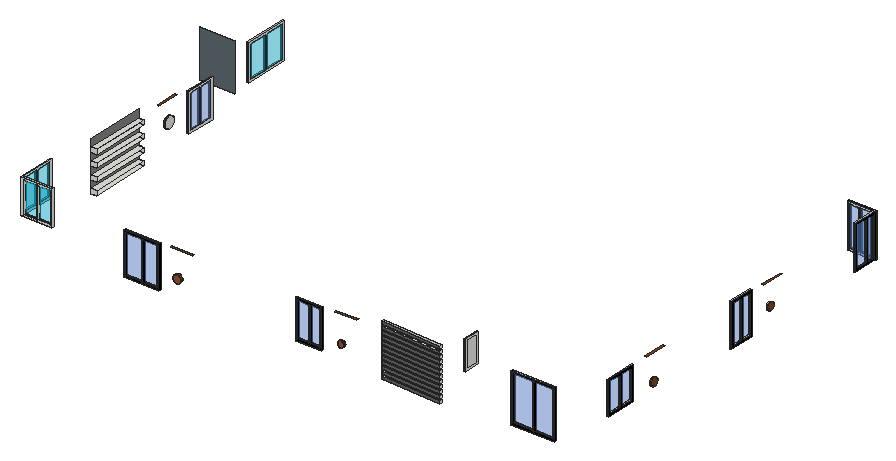
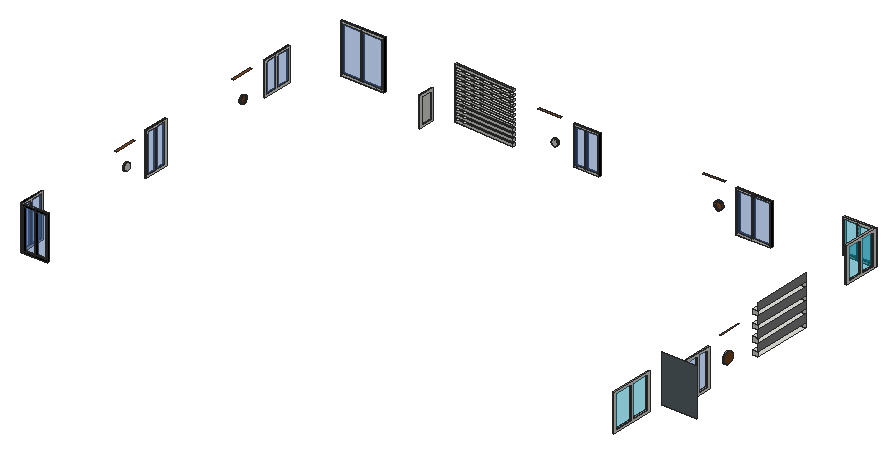
# SketchUp Ruby script. Lengths in inches.
U = 1.inch
M = Sketchup.active_model
def pt(a) = Geom::Point3d.new(a.map { |v| v * U })
def face(e, loops, mat)
  f = e.add_face(loops[0].map { |a| pt(a) })
  loops[1..].each { |l| e.add_face(l.map { |a| pt(a) }).erase! }
  f.material = f.back_material = mat if mat
  f
end
# faces: each face lists its corners as indices into pts; further lists are holes
def faces(e, pts, list, mat = nil) = list.each { |f| face(e, (f[0].is_a?(Array) ? f : [f]).map { |l| l.map { |i| pts[i] } }, mat) }
# xy, xz, yz: faces in a plane at the given z, y or x. An outline is a flat list of corners, or four numbers for a rectangle; further outlines are holes
def ring(l) = l.size == 4 ? [[l[0], l[1]], [l[2], l[1]], [l[2], l[3]], [l[0], l[3]]] : l.each_slice(2).to_a
def flat(e, list, mat, &to3) = list.each { |f| face(e, (f[0].is_a?(Array) ? f : [f]).map { |l| ring(l).map { |u, v| to3.(u, v) } }, mat) }
def xy(e, z, list, mat = nil) = flat(e, list, mat) { |x, y| [x, y, z] }
def xz(e, y, list, mat = nil) = flat(e, list, mat) { |x, z| [x, y, z] }
def yz(e, x, list, mat = nil) = flat(e, list, mat) { |y, z| [x, y, z] }
def lines(e, pts, list) = list.each { |a, b| e.add_line(pt(pts[a]), pt(pts[b])) }
# prism: a flat outline (further loops are holes) pulled along v
def prism(e, loops, v, mat = nil)
  f = face(e, loops, mat); d = Geom::Vector3d.new(v.map { |x| x * U })
  f.pushpull(f.normal.samedirection?(d) ? d.length : -d.length)
end
def box(e, o, s, mat = nil) = prism(e, [[o, [o[0] + s[0], o[1], o[2]], [o[0] + s[0], o[1] + s[1], o[2]], [o[0], o[1] + s[1], o[2]]]], [0, 0, s[2]], mat)
def at(x, y, z, deg = 0) = Geom::Transformation.translation(pt([x, y, z])) * Geom::Transformation.rotation(ORIGIN, Z_AXIS, deg.degrees)
def axes(o, x, y, z) = Geom::Transformation.new([*x, 0, *y, 0, *z, 0, *pt(o).to_a, 1])
def part(name) = M.definitions.add(name)
# library, detail: a bought-in or finely detailed component or shape, given as its bounding box
def library(name, o, s) = part(name).tap { |d| box(d.entities, o, s) }
def detail(e, o, s) = box(e.add_group.entities, o, s)
def put(e, d, t, mat = nil) = e.add_instance(d, t).tap { |i| i.material = mat if mat }
def group(e, t, mat = nil) = e.add_group.tap { |g| g.transformation = t; g.material = mat if mat }.entities
root = M.entities
M.materials.add("[0133_Gray]").color = [128, 128, 128]
M.materials.add("[0134_DimGray]").color = [105, 105, 105]
M.materials.add("[0137_Black]").color = [0, 0, 0]
M.materials.add("[Formica Speckled Grey]").color = [94, 105, 111]
M.materials.add("[Translucent Glass Blue]").color = [100, 149, 237]
M.materials["[Translucent Glass Blue]"].alpha = 0.5
M.materials.add("[Translucent Glass Tinted]").color = [8, 201, 241]
M.materials["[Translucent Glass Tinted]"].alpha = 0.48
M.materials.add("[Wood Cherry Original]").color = [152, 86, 42]
M.materials.add("[Wood Veneer 01]").color = [120, 70, 37]
xy(root,390.48,[[766.19,148.96,667.84,154.96,668.06,158.52,766.41,152.52]])
xy(root,390.84,[[249.03,155.58,306.03,158.58]])
xy(root,392.41,[[80.8125,493.7,83.8125,541.45]])
xy(root,392.87,[[83.8125,295.24,92.8125,392.06]])
xy(root,393.84,[[252.03,155.58,277.53,158.58],[280.24,155.58,303.03,158.58]],"[0137_Black]")
xy(root,394.68,[[766.19,148.96,766.41,152.52,668.06,158.52,667.84,154.96]])
xy(root,395.41,[[80.8125,496.7,83.8125,515.04],[80.8125,517.58,83.8125,538.45]])
xy(root,396.63,[[528.12,155.58,569.87,158.58]])
xy(root,396.78,[[877.02,155.58,947.52,158.58]],"[0137_Black]")
xy(root,397.73,[[766.19,148.96,667.84,154.96,668.06,158.52,766.41,152.52]])
xy(root,397.87,[[972.47,480.96,975.47,521.21]])
xy(root,399.63,[[531.12,155.58,549,158.58],[551.64,155.58,566.87,158.58]],"[0137_Black]")
xy(root,399.78,[[912.27,155.58,914.48,158.58]])
xy(root,399.78,[[880.02,155.58,912.27,158.58],[914.48,155.58,944.52,158.58]],"[0137_Black]")
xy(root,400.19,[[972.47,731.11,975.47,770.48],[931.65,770.48,972.47,773.48],[972.47,770.48,975.47,773.48]])
xy(root,400.31,[[83.8125,295.24,92.8125,392.06]])
xy(root,400.87,[[972.47,483.96,975.47,501.09],[972.47,503.31,975.47,518.21]],"[0137_Black]")
xy(root,401.93,[[766.19,148.96,766.41,152.52,668.06,158.52,667.84,154.96]])
xy(root,403.19,[[972.47,734.11,975.47,753.375],[972.47,755.28,975.47,767.48],[934.65,770.48,949.85,773.48],[952.0625,770.48,969.47,773.48]],"[0137_Black]")
xy(root,404.98,[[766.19,148.96,667.84,154.96,668.06,158.52,766.41,152.52]])
xy(root,409.18,[[766.19,148.96,766.41,152.52,668.06,158.52,667.84,154.96]])
xy(root,409.32,[[972.47,230.61,975.47,280.48]])
xy(root,412.23,[[766.19,148.96,667.84,154.96,668.06,158.52,766.41,152.52]])
xy(root,412.32,[[972.47,233.61,975.47,255.55],[972.47,258.14,975.47,277.48]],"[0137_Black]")
xy(root,412.81,[[83.8125,295.24,92.8125,392.06]])
xy(root,412.82,[[80.8125,615.71,83.8125,687.27]])
xy(root,414.22,[[763.41,201.89,766.41,227.45]])
xy(root,415.82,[[80.8125,618.71,83.8125,649.03],[80.8125,651.49,83.8125,684.27]])
xy(root,416.43,[[766.19,148.96,766.41,152.52,668.06,158.52,667.84,154.96]])
xy(root,417.22,[[763.41,204.89,766.41,224.45]])
xy(root,419.48,[[766.19,148.96,667.84,154.96,668.06,158.52,766.41,152.52]])
xy(root,420.25,[[83.8125,295.24,92.8125,392.06]])
xy(root,421.47,[[80.8125,155.58,83.8125,214.96]])
xy(root,421.66,[[83.8125,155.58,132.6875,158.58],[83.8125,158.58,132.6875,158.77]])
xy(root,423.68,[[766.19,148.96,766.41,152.52,668.06,158.52,667.84,154.96]])
xy(root,424.47,[[80.8125,161.58,83.8125,184.96],[80.8125,186.77,83.8125,211.96]])
xy(root,424.66,[[86.8125,155.58,108.25,158.58],[109.36,155.58,129.6875,158.58],[86.8125,158.58,108.25,158.77],[109.36,158.58,129.6875,158.77]])
xy(root,426.73,[[766.19,148.96,667.84,154.96,668.06,158.52,766.41,152.52]])
xy(root,430.93,[[766.19,148.96,766.41,152.52,668.06,158.52,667.84,154.96]])
xy(root,432.75,[[83.8125,295.24,92.8125,392.06]])
xy(root,433.98,[[766.19,148.96,667.84,154.96,668.06,158.52,766.41,152.52]])
xy(root,438.18,[[766.19,148.96,766.41,152.52,668.06,158.52,667.84,154.96]])
xy(root,440.19,[[83.8125,295.24,92.8125,392.06]])
xy(root,441.23,[[766.19,148.96,667.84,154.96,668.06,158.52,766.41,152.52]])
xy(root,445.43,[[766.19,148.96,766.41,152.52,668.06,158.52,667.84,154.96]])
xy(root,448.48,[[766.19,148.96,667.84,154.96,668.06,158.52,766.41,152.52]])
xy(root,450.73,[[80.8125,496.7,83.8125,515.04],[80.8125,517.58,83.8125,538.45]])
xy(root,452.68,[[766.19,148.96,766.41,152.52,668.06,158.52,667.84,154.96],[83.8125,295.24,92.8125,392.06]])
xy(root,453.73,[[80.8125,493.7,83.8125,541.45]])
xy(root,455.71,[[252.03,155.58,277.53,158.58],[280.24,155.58,303.03,158.58]],"[0137_Black]")
xy(root,455.73,[[766.19,148.96,667.84,154.96,668.06,158.52,766.41,152.52]])
xy(root,456.19,[[531.12,155.58,549,158.58],[551.64,155.58,566.87,158.58]],"[0137_Black]")
xy(root,458.71,[[249.03,155.58,306.03,158.58]],"[0137_Black]")
xy(root,458.85,[[763.41,204.89,766.41,224.45]])
xy(root,459.19,[[528.12,155.58,569.87,158.58]],"[0137_Black]")
xy(root,459.93,[[766.19,148.96,766.41,152.52,668.06,158.52,667.84,154.96]])
xy(root,460.01,[[972.47,233.61,975.47,255.55],[972.47,258.14,975.47,277.48]])
xy(root,460.06,[[80.8125,433.46,83.8125,469.46]],"[Wood Veneer 01]")
xy(root,460.13,[[83.8125,295.24,92.8125,392.06]])
xy(root,460.47,[[324.41,155.58,360.41,158.58]],"[Wood Cherry Original]")
xy(root,460.6,[[591.01,155.58,627.01,158.58]],"[Wood Cherry Original]")
xy(root,461.85,[[763.41,201.89,766.41,227.45]])
xy(root,462.87,[[972.47,545.86,975.47,581.86]],"[Wood Veneer 01]")
xy(root,462.98,[[766.19,148.96,667.84,154.96,668.06,158.52,766.41,152.52]])
xy(root,463.01,[[972.47,230.61,975.47,280.48]],"[0137_Black]")
xy(root,463.19,[[972.47,308.12,975.47,344.12]],"[Wood Veneer 01]")
xy(root,463.75,[[972.47,483.96,975.47,501.09],[972.47,503.31,975.47,518.21]],"[0137_Black]")
xy(root,466.75,[[972.47,480.96,975.47,521.21]],"[0137_Black]")
xy(root,467.18,[[766.19,148.96,766.41,152.52,668.06,158.52,667.84,154.96]])
xy(root,468.13,[[972.47,734.11,975.47,753.375],[972.47,755.28,975.47,767.48],[934.65,770.48,949.85,773.48],[952.0625,770.48,969.47,773.48]],"[0137_Black]")
xy(root,468.63,[[80.8125,618.71,83.8125,649.03],[80.8125,651.49,83.8125,684.27]])
xy(root,470.23,[[766.19,148.96,667.84,154.96,668.06,158.52,766.41,152.52]])
xz(root,152.58,[[603.27,413.39,604.58,413.5625,605.81,414.07,606.85,414.87,607.66,415.92,608.16,417.14,608.34,418.45,608.16,419.76,607.66,420.98,606.85,422.03,605.81,422.83,604.58,423.34,603.27,423.51,601.96,423.34,600.74,422.83,599.69,422.03,598.89,420.98,598.38,419.76,598.21,418.45,598.38,417.14,598.89,415.92,599.69,414.87,600.74,414.07,601.96,413.5625],[337.43,413.47,339.12,413.69,340.68,414.34,342.03,415.375,343.0625,416.72,343.71,418.29,343.93,419.97,343.71,421.65,343.0625,423.22,342.03,424.57,340.68,425.6,339.12,426.25,337.43,426.47,335.75,426.25,334.18,425.6,332.84,424.57,331.8,423.22,331.15,421.65,330.93,419.97,331.15,418.29,331.8,416.72,332.84,415.375,334.18,414.34,335.75,413.69]],"[Wood Cherry Original]")
xz(root,155.58,[[603.27,413.39,601.96,413.5625,600.74,414.07,599.69,414.87,598.89,415.92,598.38,417.14,598.21,418.45,598.38,419.76,598.89,420.98,599.69,422.03,600.74,422.83,601.96,423.34,603.27,423.51,604.58,423.34,605.81,422.83,606.85,422.03,607.66,420.98,608.16,419.76,608.34,418.45,608.16,417.14,607.66,415.92,606.85,414.87,605.81,414.07,604.58,413.5625],[[80.8125,421.47,83.8125,421.47,83.8125,421.66,132.6875,421.66,132.6875,477.85,80.8125,477.85],[86.8125,424.66,108.25,474.85],[109.36,424.66,129.6875,474.85]]])
xz(root,155.58,[[[249.03,390.84,306.03,458.71],[252.03,393.84,277.53,455.71],[280.24,393.84,303.03,455.71]],[[528.12,396.63,569.87,459.19],[531.12,399.63,549,456.19],[551.64,399.63,566.87,456.19]],[[877.02,396.78,947.52,475.53],[880.02,399.78,944.52,472.53]],[912.27,399.78,914.48,472.53]],"[0137_Black]")
xz(root,158.58,[[[249.03,390.84,306.03,458.71],[252.03,393.84,277.53,455.71],[280.24,393.84,303.03,455.71]],[[528.12,396.63,569.87,459.19],[531.12,399.63,549,456.19],[551.64,399.63,566.87,456.19]],[[877.02,396.78,947.52,475.53],[880.02,399.78,944.52,472.53]],[912.27,399.78,914.48,472.53],[[83.8125,421.66,132.6875,477.85],[86.8125,424.66,108.25,474.85],[109.36,424.66,129.6875,474.85]]])
xz(root,158.58,[[252.03,393.84,277.53,455.71],[280.24,393.84,303.03,455.71],[531.12,399.63,549,456.19],[551.64,399.63,566.87,456.19],[880.02,399.78,912.27,472.53],
  [914.48,399.78,944.52,472.53]],"[Translucent Glass Blue]")
xz(root,158.58,[[86.8125,424.66,108.25,474.85],[109.36,424.66,129.6875,474.85]],"[Translucent Glass Tinted]")
xz(root,158.77,[[[83.8125,421.66,132.6875,477.85],[86.8125,424.66,108.25,474.85],[109.36,424.66,129.6875,474.85]]])
xz(root,161.58,[[80.8125,424.47,83.8125,474.85]])
xz(root,184.96,[[80.8125,424.47,83.8125,474.85]])
xz(root,186.77,[[80.8125,424.47,83.8125,474.85]])
xz(root,201.89,[[763.41,414.22,766.41,461.85]])
xz(root,204.89,[[763.41,417.22,766.41,458.85]])
xz(root,211.96,[[80.8125,424.47,83.8125,474.85]])
xz(root,214.96,[[80.8125,421.47,83.8125,477.85]])
xz(root,224.45,[[763.41,417.22,766.41,458.85]])
xz(root,227.45,[[763.41,414.22,766.41,461.85]])
xz(root,230.61,[[972.47,409.32,975.47,463.01]],"[0137_Black]")
xz(root,233.61,[[972.47,412.32,975.47,460.01]],"[0137_Black]")
xz(root,255.55,[[972.47,412.32,975.47,460.01]],"[0137_Black]")
xz(root,258.14,[[972.47,412.32,975.47,460.01]],"[0137_Black]")
xz(root,277.48,[[972.47,412.32,975.47,460.01]],"[0137_Black]")
xz(root,280.48,[[972.47,409.32,975.47,463.01]],"[0137_Black]")
xz(root,295.24,[[83.8125,392.87,92.8125,400.31],[83.8125,412.81,92.8125,420.25],[83.8125,432.75,92.8125,440.19],[83.8125,452.68,92.8125,460.13]])
xz(root,392.06,[[83.8125,392.87,92.8125,400.31],[83.8125,412.81,92.8125,420.25],[83.8125,432.75,92.8125,440.19],[83.8125,452.68,92.8125,460.13]])
xz(root,480.96,[[972.47,397.87,975.47,466.75]],"[0137_Black]")
xz(root,483.96,[[972.47,400.87,975.47,463.75]],"[0137_Black]")
xz(root,493.7,[[80.8125,392.41,83.8125,453.73]])
xz(root,496.7,[[80.8125,395.41,83.8125,450.73]])
xz(root,501.09,[[972.47,400.87,975.47,463.75]],"[0137_Black]")
xz(root,503.31,[[972.47,400.87,975.47,463.75]],"[0137_Black]")
xz(root,515.04,[[80.8125,395.41,83.8125,450.73]])
xz(root,517.58,[[80.8125,395.41,83.8125,450.73]])
xz(root,518.21,[[972.47,400.87,975.47,463.75]],"[0137_Black]")
xz(root,521.21,[[972.47,397.87,975.47,466.75]],"[0137_Black]")
xz(root,538.45,[[80.8125,395.41,83.8125,450.73]])
xz(root,541.45,[[80.8125,392.41,83.8125,453.73]])
xz(root,587.65,[[26.03,409.42,83.8125,486.18]],"[Formica Speckled Grey]")
xz(root,615.71,[[80.8125,412.82,83.8125,471.63]])
xz(root,618.71,[[80.8125,415.82,83.8125,468.63]])
xz(root,649.03,[[80.8125,415.82,83.8125,468.63]])
xz(root,651.49,[[80.8125,415.82,83.8125,468.63]])
xz(root,684.27,[[80.8125,415.82,83.8125,468.63]])
xz(root,687.27,[[80.8125,412.82,83.8125,471.63]])
xz(root,731.11,[[972.47,400.19,975.47,471.13]])
xz(root,734.11,[[972.47,403.19,975.47,468.13]],"[0137_Black]")
xz(root,753.375,[[972.47,403.19,975.47,468.13]],"[0137_Black]")
xz(root,755.28,[[972.47,403.19,975.47,468.13]],"[0137_Black]")
xz(root,767.48,[[972.47,403.19,975.47,468.13]],"[0137_Black]")
xz(root,770.48,[[[931.65,400.19,972.47,471.13],[952.0625,403.19,969.47,468.13],[934.65,403.19,949.85,468.13]],[972.47,400.19,975.47,471.13]])
xz(root,770.48,[[934.65,403.19,949.85,468.13],[952.0625,403.19,969.47,468.13]],"[Translucent Glass Blue]")
xz(root,773.48,[[[931.65,400.19,972.47,471.13],[952.0625,403.19,969.47,468.13],[934.65,403.19,949.85,468.13]],[972.47,400.19,975.47,471.13]],"[0137_Black]")
yz(root,77.8125,[[458.74,414.24,456.41,414.54,454.24,415.44,452.375,416.87,450.95,418.74,450.05,420.91,449.74,423.24,450.05,425.57,450.95,427.74,452.375,429.6,454.24,431.03,456.41,431.93,458.74,432.24,461.07,431.93,463.24,431.03,465.1,429.6,466.53,427.74,467.43,425.57,467.74,423.24,467.43,420.91,466.53,418.74,465.1,416.87,463.24,415.44,461.07,414.54]],"[Wood Veneer 01]")
yz(root,80.8125,[[[493.7,392.41,541.45,453.73],[517.58,395.41,538.45,450.73],[496.7,395.41,515.04,450.73]],[[615.71,412.82,687.27,471.63],[651.49,415.82,684.27,468.63],[618.71,415.82,649.03,468.63]],[458.74,414.24,461.07,414.54,463.24,415.44,465.1,416.87,466.53,418.74,467.43,420.91,467.74,423.24,467.43,425.57,466.53,427.74,465.1,429.6,463.24,431.03,461.07,431.93,458.74,432.24,456.41,431.93,454.24,431.03,452.375,429.6,450.95,427.74,450.05,425.57,449.74,423.24,450.05,420.91,450.95,418.74,452.375,416.87,454.24,415.44,456.41,414.54],[[155.58,421.47,214.96,477.85],[186.77,424.47,211.96,474.85],[161.58,424.47,184.96,474.85]]])
yz(root,83.8125,[[[493.7,392.41,541.45,453.73],[517.58,395.41,538.45,450.73],[496.7,395.41,515.04,450.73]],[[615.71,412.82,687.27,471.63],[651.49,415.82,684.27,468.63],[618.71,415.82,649.03,468.63]],[155.58,421.47,158.58,421.66],[[158.58,421.47,214.96,421.47,214.96,477.85,158.77,477.85,158.77,421.66,158.58,421.66],[186.77,424.47,211.96,474.85],[161.58,424.47,184.96,474.85]],[158.58,421.66,158.77,477.85]])
yz(root,83.8125,[[295.24,400.31,392.06,412.81],[295.24,420.25,392.06,432.75],[295.24,440.19,392.06,452.68],[295.24,460.13,392.06,472.62]],"[0133_Gray]")
yz(root,83.8125,[[496.7,395.41,515.04,450.73],[517.58,395.41,538.45,450.73]],"[Translucent Glass Blue]")
yz(root,83.8125,[[618.71,415.82,649.03,468.63],[651.49,415.82,684.27,468.63],[161.58,424.47,184.96,474.85],[186.77,424.47,211.96,474.85]],"[Translucent Glass Tinted]")
yz(root,86.8125,[[155.58,424.66,158.58,474.85],[158.58,424.66,158.77,474.85]])
yz(root,108.25,[[155.58,424.66,158.58,474.85],[158.58,424.66,158.77,474.85]])
yz(root,109.36,[[155.58,424.66,158.58,474.85],[158.58,424.66,158.77,474.85]])
yz(root,129.6875,[[155.58,424.66,158.58,474.85],[158.58,424.66,158.77,474.85]])
yz(root,132.6875,[[155.58,421.66,158.58,477.85],[158.58,421.66,158.77,477.85]])
yz(root,249.03,[[155.58,390.84,158.58,458.71]],"[0137_Black]")
yz(root,252.03,[[155.58,393.84,158.58,455.71]],"[0137_Black]")
yz(root,277.53,[[155.58,393.84,158.58,455.71]],"[0137_Black]")
yz(root,280.24,[[155.58,393.84,158.58,455.71]],"[0137_Black]")
yz(root,303.03,[[155.58,393.84,158.58,455.71]],"[0137_Black]")
yz(root,306.03,[[155.58,390.84,158.58,458.71]],"[0137_Black]")
yz(root,528.12,[[155.58,396.63,158.58,459.19]],"[0137_Black]")
yz(root,531.12,[[155.58,399.63,158.58,456.19]],"[0137_Black]")
yz(root,549,[[155.58,399.63,158.58,456.19]],"[0137_Black]")
yz(root,551.64,[[155.58,399.63,158.58,456.19]],"[0137_Black]")
yz(root,566.87,[[155.58,399.63,158.58,456.19]],"[0137_Black]")
yz(root,569.87,[[155.58,396.63,158.58,459.19]],"[0137_Black]")
yz(root,763.41,[[[201.89,414.22,227.45,461.85],[204.89,417.22,224.45,458.85]]])
yz(root,766.41,[[[201.89,414.22,227.45,461.85],[204.89,417.22,224.45,458.85]],[204.89,417.22,224.45,458.85]])
yz(root,877.02,[[155.58,396.78,158.58,475.53]],"[0137_Black]")
yz(root,880.02,[[155.58,399.78,158.58,472.53]],"[0137_Black]")
yz(root,912.27,[[155.58,399.78,158.58,472.53]],"[0137_Black]")
yz(root,914.48,[[155.58,399.78,158.58,472.53]],"[0137_Black]")
yz(root,931.65,[[770.48,400.19,773.48,471.13]],"[0137_Black]")
yz(root,934.65,[[770.48,403.19,773.48,468.13]],"[0137_Black]")
yz(root,944.52,[[155.58,399.78,158.58,472.53]],"[0137_Black]")
yz(root,947.52,[[155.58,396.78,158.58,475.53]],"[0137_Black]")
yz(root,949.85,[[770.48,403.19,773.48,468.13]],"[0137_Black]")
yz(root,952.0625,[[770.48,403.19,773.48,468.13]],"[0137_Black]")
yz(root,969.47,[[770.48,403.19,773.48,468.13]],"[0137_Black]")
yz(root,972.47,[[[480.96,397.87,521.21,466.75],[483.96,400.87,501.09,463.75],[503.31,400.87,518.21,463.75]],[[731.11,400.19,770.48,471.13],[734.11,403.19,753.375,468.13],[755.28,403.19,767.48,468.13]],[770.48,400.19,773.48,471.13],[[230.61,409.32,280.48,463.01],[233.61,412.32,255.55,460.01],[258.14,412.32,277.48,460.01]]])
yz(root,972.47,[[483.96,400.87,501.09,463.75],[503.31,400.87,518.21,463.75],[734.11,403.19,753.375,468.13],[755.28,403.19,767.48,468.13],[233.61,412.32,255.55,460.01],
  [258.14,412.32,277.48,460.01]],"[Translucent Glass Blue]")
yz(root,975.47,[[556.25,422.52,554.76,422.71,553.38,423.29,552.1875,424.2,551.27,425.39,550.7,426.78,550.5,428.27,550.7,429.76,551.27,431.14,552.1875,432.33,553.38,433.25,554.76,433.82,556.25,434.02,557.74,433.82,559.13,433.25,560.32,432.33,561.23,431.14,561.81,429.76,562,428.27,561.81,426.78,561.23,425.39,560.32,424.2,559.13,423.29,557.74,422.71]])
yz(root,975.47,[[[480.96,397.87,521.21,466.75],[483.96,400.87,501.09,463.75],[503.31,400.87,518.21,463.75]],[[731.11,400.19,770.48,471.13],[734.11,403.19,753.375,468.13],[755.28,403.19,767.48,468.13]],[770.48,400.19,773.48,471.13],[[230.61,409.32,280.48,463.01],[233.61,412.32,255.55,460.01],[258.14,412.32,277.48,460.01]]],"[0137_Black]")
yz(root,978.47,[[319.91,416.2,321.5,416.41,322.98,417.02,324.25,418,325.22,419.26,325.83,420.74,326.04,422.33,325.83,423.91,325.22,425.39,324.25,426.66,322.98,427.63,321.5,428.24,319.91,428.45,318.33,428.24,316.85,427.63,315.58,426.66,314.61,425.39,314,423.91,313.79,422.33,314,420.74,314.61,419.26,315.58,418,316.85,417.02,318.33,416.41],[556.25,422.52,557.74,422.71,559.13,423.29,560.32,424.2,561.23,425.39,561.81,426.78,562,428.27,561.81,429.76,561.23,431.14,560.32,432.33,559.13,433.25,557.74,433.82,556.25,434.02,554.76,433.82,553.38,433.25,552.1875,432.33,551.27,431.14,550.7,429.76,550.5,428.27,550.7,426.78,551.27,425.39,552.1875,424.2,553.38,423.29,554.76,422.71]],"[Wood Veneer 01]")
p = [[766.19,148.96,394.68],[667.84,154.96,394.68],[667.84,154.96,390.48],[766.19,148.96,390.48],[766.41,152.52,390.48],[766.41,152.52,394.68],
  [668.06,158.52,394.68],[668.06,158.52,390.48],[766.19,148.96,401.93],[667.84,154.96,401.93],[667.84,154.96,397.73],[766.19,148.96,397.73],
  [766.41,152.52,397.73],[766.41,152.52,401.93],[668.06,158.52,401.93],[668.06,158.52,397.73],[766.19,148.96,409.18],[667.84,154.96,409.18],
  [667.84,154.96,404.98],[766.19,148.96,404.98],[766.41,152.52,404.98],[766.41,152.52,409.18],[668.06,158.52,409.18],[668.06,158.52,404.98],
  [766.19,148.96,416.43],[667.84,154.96,416.43],[667.84,154.96,412.23],[766.19,148.96,412.23],[766.41,152.52,412.23],[766.41,152.52,416.43],
  [668.06,158.52,416.43],[668.06,158.52,412.23],[601.96,155.58,413.5625],[603.27,155.58,413.39],[603.27,152.58,413.39],[601.96,152.58,413.5625],
  [604.58,155.58,413.5625],[604.58,152.58,413.5625],[335.75,155.58,413.69],[337.43,155.58,413.47],[337.43,152.58,413.47],[335.75,152.58,413.69],
  [339.12,155.58,413.69],[339.12,152.58,413.69],[600.74,155.58,414.07],[600.74,152.58,414.07],[605.81,155.58,414.07],[605.81,152.58,414.07],
  [334.18,155.58,414.34],[334.18,152.58,414.34],[340.68,155.58,414.34],[340.68,152.58,414.34],[599.69,155.58,414.87],[599.69,152.58,414.87],
  [606.85,155.58,414.87],[606.85,152.58,414.87],[80.8125,458.74,414.24],[80.8125,456.41,414.54],[77.8125,456.41,414.54],[77.8125,458.74,414.24],
  [80.8125,461.07,414.54],[77.8125,461.07,414.54],[332.84,155.58,415.375],[332.84,152.58,415.375],[342.03,155.58,415.375],[342.03,152.58,415.375],
  [80.8125,454.24,415.44],[77.8125,454.24,415.44],[80.8125,463.24,415.44],[77.8125,463.24,415.44],[598.89,155.58,415.92],[598.89,152.58,415.92],
  [607.66,155.58,415.92],[607.66,152.58,415.92],[331.8,155.58,416.72],[331.8,152.58,416.72],[343.0625,155.58,416.72],[343.0625,152.58,416.72],
  [80.8125,452.375,416.87],[77.8125,452.375,416.87],[80.8125,465.1,416.87],[77.8125,465.1,416.87],[598.38,155.58,417.14],[598.38,152.58,417.14],
  [608.16,155.58,417.14],[608.16,152.58,417.14],[975.47,318.33,416.41],[975.47,319.91,416.2],[978.47,319.91,416.2],[978.47,318.33,416.41],
  [975.47,321.5,416.41],[978.47,321.5,416.41],[975.47,316.85,417.02],[978.47,316.85,417.02],[975.47,322.98,417.02],[978.47,322.98,417.02],
  [331.15,155.58,418.29],[331.15,152.58,418.29],[343.71,155.58,418.29],[343.71,152.58,418.29],[80.8125,450.95,418.74],[77.8125,450.95,418.74],
  [80.8125,466.53,418.74],[77.8125,466.53,418.74],[975.47,315.58,418],[978.47,315.58,418],[975.47,324.25,418],[978.47,324.25,418],
  [598.21,155.58,418.45],[598.21,152.58,418.45],[608.34,155.58,418.45],[608.34,152.58,418.45],[975.47,314.61,419.26],[978.47,314.61,419.26],
  [975.47,325.22,419.26],[978.47,325.22,419.26],[330.93,155.58,419.97],[330.93,152.58,419.97],[343.93,155.58,419.97],[343.93,152.58,419.97],
  [598.38,155.58,419.76],[598.38,152.58,419.76],[608.16,155.58,419.76],[608.16,152.58,419.76],[80.8125,450.05,420.91],[77.8125,450.05,420.91],
  [80.8125,467.43,420.91],[77.8125,467.43,420.91],[975.47,314,420.74],[978.47,314,420.74],[975.47,325.83,420.74],[978.47,325.83,420.74],
  [766.19,148.96,423.68],[667.84,154.96,423.68],[667.84,154.96,419.48],[766.19,148.96,419.48],[766.41,152.52,419.48],[766.41,152.52,423.68],
  [668.06,158.52,423.68],[668.06,158.52,419.48],[598.89,155.58,420.98],[598.89,152.58,420.98],[607.66,155.58,420.98],[607.66,152.58,420.98],
  [331.15,155.58,421.65],[331.15,152.58,421.65],[343.71,155.58,421.65],[343.71,152.58,421.65],[975.47,313.79,422.33],[978.47,313.79,422.33],
  [975.47,326.04,422.33],[978.47,326.04,422.33],[80.8125,449.74,423.24],[77.8125,449.74,423.24],[80.8125,467.74,423.24],[77.8125,467.74,423.24],
  [599.69,155.58,422.03],[599.69,152.58,422.03],[606.85,155.58,422.03],[606.85,152.58,422.03],[331.8,155.58,423.22],[331.8,152.58,423.22],
  [343.0625,155.58,423.22],[343.0625,152.58,423.22],[600.74,155.58,422.83],[600.74,152.58,422.83],[605.81,155.58,422.83],[605.81,152.58,422.83],
  [975.47,314,423.91],[978.47,314,423.91],[975.47,325.83,423.91],[978.47,325.83,423.91],[975.47,554.76,422.71],[975.47,556.25,422.52],
  [978.47,556.25,422.52],[978.47,554.76,422.71],[975.47,557.74,422.71],[978.47,557.74,422.71],[975.47,553.38,423.29],[978.47,553.38,423.29],
  [975.47,559.13,423.29],[978.47,559.13,423.29],[601.96,155.58,423.34],[601.96,152.58,423.34],[604.58,155.58,423.34],[604.58,152.58,423.34],
  [332.84,155.58,424.57],[332.84,152.58,424.57],[342.03,155.58,424.57],[342.03,152.58,424.57],[80.8125,450.05,425.57],[77.8125,450.05,425.57],
  [80.8125,467.43,425.57],[77.8125,467.43,425.57],[603.27,155.58,423.51],[603.27,152.58,423.51],[975.47,552.1875,424.2],[978.47,552.1875,424.2],
  [975.47,560.32,424.2],[978.47,560.32,424.2],[975.47,314.61,425.39],[978.47,314.61,425.39],[975.47,325.22,425.39],[978.47,325.22,425.39],
  [975.47,551.27,425.39],[978.47,551.27,425.39],[975.47,561.23,425.39],[978.47,561.23,425.39],[334.18,155.58,425.6],[334.18,152.58,425.6],
  [340.68,155.58,425.6],[340.68,152.58,425.6],[975.47,315.58,426.66],[978.47,315.58,426.66],[975.47,324.25,426.66],[978.47,324.25,426.66],
  [975.47,550.7,426.78],[978.47,550.7,426.78],[975.47,561.81,426.78],[978.47,561.81,426.78],[335.75,155.58,426.25],[335.75,152.58,426.25],
  [339.12,155.58,426.25],[339.12,152.58,426.25],[80.8125,450.95,427.74],[77.8125,450.95,427.74],[80.8125,466.53,427.74],[77.8125,466.53,427.74],
  [337.43,155.58,426.47],[337.43,152.58,426.47],[766.19,148.96,430.93],[667.84,154.96,430.93],[667.84,154.96,426.73],[766.19,148.96,426.73],
  [766.41,152.52,426.73],[766.41,152.52,430.93],[668.06,158.52,430.93],[668.06,158.52,426.73],[975.47,316.85,427.63],[978.47,316.85,427.63],
  [975.47,322.98,427.63],[978.47,322.98,427.63],[975.47,550.5,428.27],[978.47,550.5,428.27],[975.47,562,428.27],[978.47,562,428.27],
  [975.47,318.33,428.24],[978.47,318.33,428.24],[975.47,321.5,428.24],[978.47,321.5,428.24],[80.8125,452.375,429.6],[77.8125,452.375,429.6],
  [80.8125,465.1,429.6],[77.8125,465.1,429.6],[975.47,319.91,428.45],[978.47,319.91,428.45],[975.47,550.7,429.76],[978.47,550.7,429.76],
  [975.47,561.81,429.76],[978.47,561.81,429.76],[80.8125,454.24,431.03],[77.8125,454.24,431.03],[80.8125,463.24,431.03],[77.8125,463.24,431.03],
  [975.47,551.27,431.14],[978.47,551.27,431.14],[975.47,561.23,431.14],[978.47,561.23,431.14],[80.8125,456.41,431.93],[77.8125,456.41,431.93],
  [80.8125,461.07,431.93],[77.8125,461.07,431.93],[975.47,552.1875,432.33],[978.47,552.1875,432.33],[975.47,560.32,432.33],[978.47,560.32,432.33],
  [80.8125,458.74,432.24],[77.8125,458.74,432.24],[975.47,553.38,433.25],[978.47,553.38,433.25],[975.47,559.13,433.25],[978.47,559.13,433.25],
  [975.47,554.76,433.82],[978.47,554.76,433.82],[975.47,557.74,433.82],[978.47,557.74,433.82],[975.47,556.25,434.02],[978.47,556.25,434.02],
  [766.19,148.96,438.18],[667.84,154.96,438.18],[667.84,154.96,433.98],[766.19,148.96,433.98],[766.41,152.52,433.98],[766.41,152.52,438.18],
  [668.06,158.52,438.18],[668.06,158.52,433.98],[766.19,148.96,445.43],[667.84,154.96,445.43],[667.84,154.96,441.23],[766.19,148.96,441.23],
  [766.41,152.52,441.23],[766.41,152.52,445.43],[668.06,158.52,445.43],[668.06,158.52,441.23],[766.19,148.96,452.68],[667.84,154.96,452.68],
  [667.84,154.96,448.48],[766.19,148.96,448.48],[766.41,152.52,448.48],[766.41,152.52,452.68],[668.06,158.52,452.68],[668.06,158.52,448.48],
  [766.19,148.96,459.93],[667.84,154.96,459.93],[667.84,154.96,455.73],[766.19,148.96,455.73],[766.41,152.52,455.73],[766.41,152.52,459.93],
  [668.06,158.52,459.93],[668.06,158.52,455.73],[766.19,148.96,467.18],[667.84,154.96,467.18],[667.84,154.96,462.98],[766.19,148.96,462.98],
  [766.41,152.52,462.98],[766.41,152.52,467.18],[668.06,158.52,467.18],[668.06,158.52,462.98],[766.19,148.96,474.43],[667.84,154.96,474.43],
  [667.84,154.96,470.23],[766.19,148.96,470.23],[766.41,152.52,470.23],[766.41,152.52,474.43],[668.06,158.52,474.43],[668.06,158.52,470.23],
  [83.8125,158.58,421.66],[80.8125,158.58,421.66],[83.8125,158.77,421.66],[80.8125,158.77,421.66]]
faces(root,p,[[0,1,2,3],[8,9,10,11],[16,17,18,19],[24,25,26,27],[132,133,134,135],[230,231,232,233],[288,289,290,291],[296,297,298,299],
  [304,305,306,307],[312,313,314,315],[320,321,322,323],[328,329,330,331]],"[0134_DimGray]")
faces(root,p,[[4,5,0,3],[6,5,4,7],[6,7,2,1],[12,13,8,11],[14,13,12,15],[14,15,10,9],[20,21,16,19],[22,21,20,23],
  [22,23,18,17],[28,29,24,27],[30,29,28,31],[30,31,26,25],[136,137,132,135],[138,137,136,139],[138,139,134,133],[234,235,230,233],
  [236,235,234,237],[236,237,232,231],[292,293,288,291],[294,293,292,295],[294,295,290,289],[300,301,296,299],[302,301,300,303],[302,303,298,297],
  [308,309,304,307],[310,309,308,311],[310,311,306,305],[316,317,312,315],[318,317,316,319],[318,319,314,313],[324,325,320,323],[326,325,324,327],
  [326,327,322,321],[332,333,328,331],[334,333,332,335],[334,335,330,329]])
faces(root,p,[[32,33,34,35],[33,36,37,34],[38,39,40,41],[39,42,43,40],[44,32,35,45],[36,46,47,37],[48,38,41,49],[42,50,51,43],
  [52,44,45,53],[46,54,55,47],[62,48,49,63],[50,64,65,51],[70,52,53,71],[54,72,73,55],[74,62,63,75],[64,76,77,65],
  [82,70,71,83],[72,84,85,73],[96,74,75,97],[76,98,99,77],[108,82,83,109],[84,110,111,85],[116,96,97,117],[98,118,119,99],
  [120,108,109,121],[110,122,123,111],[140,120,121,141],[122,142,143,123],[144,116,117,145],[118,146,147,119],[156,140,141,157],[142,158,159,143],
  [160,144,145,161],[146,162,163,147],[164,156,157,165],[158,166,167,159],[182,164,165,183],[166,184,185,167],[186,160,161,187],[162,188,189,163],
  [194,182,183,195],[184,194,195,185],[208,186,187,209],[188,210,211,189],[220,208,209,221],[210,222,223,211],[228,220,221,229],[222,228,229,223]],"[Wood Cherry Original]")
faces(root,p,[[56,57,58,59],[60,56,59,61],[57,66,67,58],[68,60,61,69],[66,78,79,67],[80,68,69,81],[86,87,88,89],[87,90,91,88],
  [92,86,89,93],[90,94,95,91],[78,100,101,79],[102,80,81,103],[104,92,93,105],[94,106,107,95],[112,104,105,113],[106,114,115,107],
  [100,124,125,101],[126,102,103,127],[128,112,113,129],[114,130,131,115],[148,128,129,149],[130,150,151,131],[124,152,153,125],[154,126,127,155],
  [168,148,149,169],[150,170,171,151],[172,173,174,175],[173,176,177,174],[178,172,175,179],[176,180,181,177],[152,190,191,153],[192,154,155,193],
  [196,178,179,197],[180,198,199,181],[200,168,169,201],[170,202,203,171],[204,196,197,205],[198,206,207,199],[212,200,201,213],[202,214,215,203],
  [216,204,205,217],[206,218,219,207],[190,224,225,191],[226,192,193,227],[238,212,213,239],[214,240,241,215],[242,216,217,243],[218,244,245,219],
  [246,238,239,247],[240,248,249,241],[224,250,251,225],[252,226,227,253],[254,246,247,255],[248,254,255,249],[256,242,243,257],[244,258,259,245],
  [250,260,261,251],[262,252,253,263],[264,256,257,265],[258,266,267,259],[260,268,269,261],[270,262,263,271],[272,264,265,273],[266,274,275,267],
  [268,276,277,269],[276,270,271,277],[278,272,273,279],[274,280,281,275],[282,278,279,283],[280,284,285,281],[286,282,283,287],[284,286,287,285]],"[Wood Veneer 01]")
lines(root,p,[[336,337],[338,339]])
